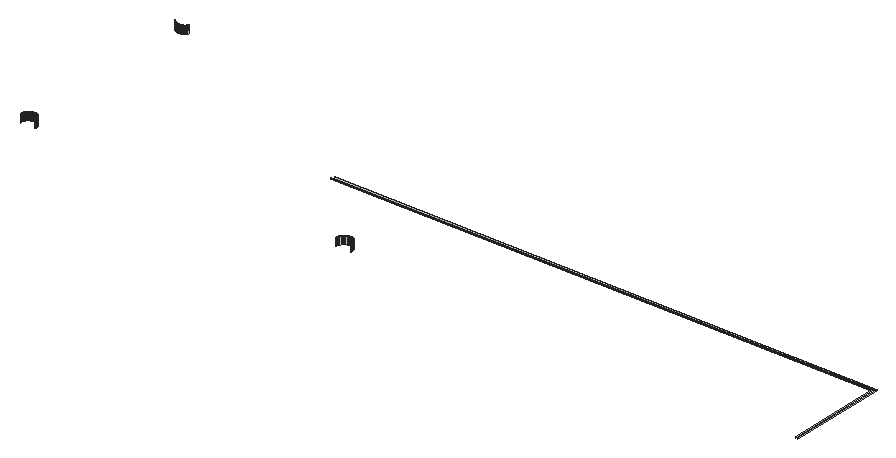
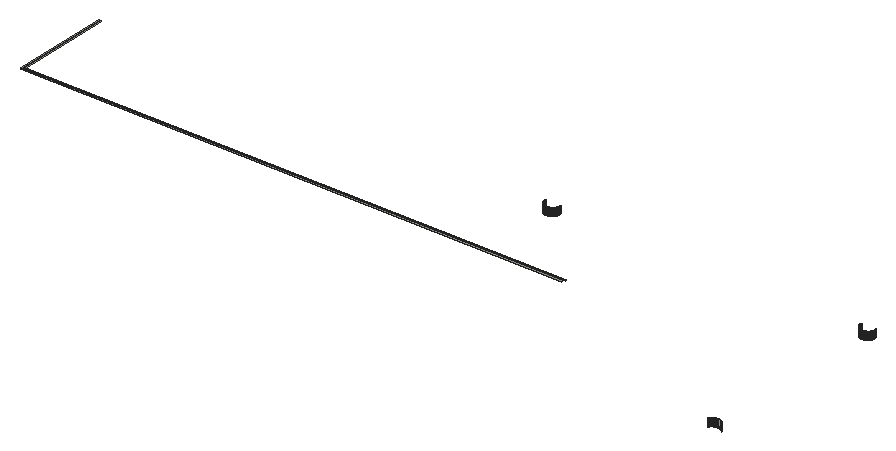
# SketchUp Ruby script. Lengths in inches.
U = 1.inch
M = Sketchup.active_model
def pt(a) = Geom::Point3d.new(a.map { |v| v * U })
def face(e, loops, mat)
  f = e.add_face(loops[0].map { |a| pt(a) })
  loops[1..].each { |l| e.add_face(l.map { |a| pt(a) }).erase! }
  f.material = f.back_material = mat if mat
  f
end
# faces: each face lists its corners as indices into pts; further lists are holes
def faces(e, pts, list, mat = nil) = list.each { |f| face(e, (f[0].is_a?(Array) ? f : [f]).map { |l| l.map { |i| pts[i] } }, mat) }
# xy, xz, yz: faces in a plane at the given z, y or x. An outline is a flat list of corners, or four numbers for a rectangle; further outlines are holes
def ring(l) = l.size == 4 ? [[l[0], l[1]], [l[2], l[1]], [l[2], l[3]], [l[0], l[3]]] : l.each_slice(2).to_a
def flat(e, list, mat, &to3) = list.each { |f| face(e, (f[0].is_a?(Array) ? f : [f]).map { |l| ring(l).map { |u, v| to3.(u, v) } }, mat) }
def xy(e, z, list, mat = nil) = flat(e, list, mat) { |x, y| [x, y, z] }
def xz(e, y, list, mat = nil) = flat(e, list, mat) { |x, z| [x, y, z] }
def yz(e, x, list, mat = nil) = flat(e, list, mat) { |y, z| [x, y, z] }
def lines(e, pts, list) = list.each { |a, b| e.add_line(pt(pts[a]), pt(pts[b])) }
# prism: a flat outline (further loops are holes) pulled along v
def prism(e, loops, v, mat = nil)
  f = face(e, loops, mat); d = Geom::Vector3d.new(v.map { |x| x * U })
  f.pushpull(f.normal.samedirection?(d) ? d.length : -d.length)
end
def box(e, o, s, mat = nil) = prism(e, [[o, [o[0] + s[0], o[1], o[2]], [o[0] + s[0], o[1] + s[1], o[2]], [o[0], o[1] + s[1], o[2]]]], [0, 0, s[2]], mat)
def at(x, y, z, deg = 0) = Geom::Transformation.translation(pt([x, y, z])) * Geom::Transformation.rotation(ORIGIN, Z_AXIS, deg.degrees)
def axes(o, x, y, z) = Geom::Transformation.new([*x, 0, *y, 0, *z, 0, *pt(o).to_a, 1])
def part(name) = M.definitions.add(name)
# library, detail: a bought-in or finely detailed component or shape, given as its bounding box
def library(name, o, s) = part(name).tap { |d| box(d.entities, o, s) }
def detail(e, o, s) = box(e.add_group.entities, o, s)
def put(e, d, t, mat = nil) = e.add_instance(d, t).tap { |i| i.material = mat if mat }
def group(e, t, mat = nil) = e.add_group.tap { |g| g.transformation = t; g.material = mat if mat }.entities
root = M.entities
M.materials.add("0027 AP L140 CRUSHED ICE").color = [241, 233, 217]
xz(root,261,[[59.84,120,59.92,123],[59.92,120,60,123],[60,120,60.08,123],[60.08,120,60.16,123],[185.84,120,185.92,123],
  [185.92,120,186,123],[186,120,186.08,123],[186.08,120,186.16,123]],"0027 AP L140 CRUSHED ICE")
xz(root,290,[[155,120,371,120.5]],"0027 AP L140 CRUSHED ICE")
xz(root,291,[[156,120,372,120.5]],"0027 AP L140 CRUSHED ICE")
xz(root,333,[[59.84,120,59.92,123],[59.92,120,60,123],[60,120,60.08,123],[60.08,120,60.16,123]],"0027 AP L140 CRUSHED ICE")
yz(root,57,[[257.84,120,257.92,123],[257.92,120,258,123],[258,120,258.08,123],[258.08,120,258.16,123]],"0027 AP L140 CRUSHED ICE")
yz(root,63,[[257.84,120,257.92,123],[257.92,120,258,123],[258,120,258.08,123],[258.08,120,258.16,123]],"0027 AP L140 CRUSHED ICE")
yz(root,183,[[257.84,120,257.92,123],[257.92,120,258,123],[258,120,258.08,123],[258.08,120,258.16,123]],"0027 AP L140 CRUSHED ICE")
yz(root,189,[[257.84,120,257.92,123],[257.92,120,258,123],[258,120,258.08,123],[258.08,120,258.16,123]],"0027 AP L140 CRUSHED ICE")
yz(root,371,[[252,120,290,120.5]],"0027 AP L140 CRUSHED ICE")
yz(root,372,[[252,120,291,120.5]],"0027 AP L140 CRUSHED ICE")
p = [[62.98,257.6875,120],[62.97,257.61,120],[62.97,257.61,123],[62.98,257.6875,123],[57.02,257.6875,120],[57.01,257.76,120],
  [57.01,257.76,123],[57.02,257.6875,123],[62.99,257.76,120],[62.99,257.76,123],[183.02,257.6875,120],[183.01,257.76,120],
  [183.01,257.76,123],[183.02,257.6875,123],[188.99,257.76,120],[188.98,257.6875,120],[188.98,257.6875,123],[188.99,257.76,123],
  [57,257.84,120],[57,257.84,123],[63,257.84,120],[63,257.84,123],[183,257.84,120],[183,257.84,123],
  [189,257.84,120],[189,257.84,123],[57,258.16,120],[57.01,258.24,120],[57.01,258.24,123],[57,258.16,123],
  [57.02,258.3125,120],[57.02,258.3125,123],[62.99,258.24,120],[63,258.16,120],[63,258.16,123],[62.99,258.24,123],
  [62.98,258.3125,120],[62.98,258.3125,123],[183,258.16,120],[183.01,258.24,120],[183.01,258.24,123],[183,258.16,123],
  [183.02,258.3125,120],[183.02,258.3125,123],[188.99,258.24,120],[189,258.16,120],[189,258.16,123],[188.99,258.24,123],
  [188.98,258.3125,120],[188.98,258.3125,123],[57.03,258.39,120],[57.03,258.39,123],[62.97,258.39,120],[62.97,258.39,123],
  [183.03,258.39,120],[183.03,258.39,123],[188.97,258.39,120],[188.97,258.39,123],[57.04,258.47,120],[57.04,258.47,123],
  [62.96,258.47,120],[62.96,258.47,123],[183.04,258.47,120],[183.04,258.47,123],[188.96,258.47,120],[188.96,258.47,123],
  [57.05,258.55,120],[57.05,258.55,123],[57.07,258.625,120],[57.07,258.625,123],[62.95,258.55,120],[62.95,258.55,123],
  [62.93,258.625,120],[62.93,258.625,123],[183.05,258.55,120],[183.05,258.55,123],[183.07,258.625,120],[183.07,258.625,123],
  [188.95,258.55,120],[188.95,258.55,123],[188.93,258.625,120],[188.93,258.625,123],[57.08,258.7,120],[57.08,258.7,123],
  [62.92,258.7,120],[62.92,258.7,123],[183.08,258.7,120],[183.08,258.7,123],[188.92,258.7,120],[188.92,258.7,123],
  [57.1,258.78,120],[57.1,258.78,123],[62.9,258.78,120],[62.9,258.78,123],[183.1,258.78,120],[183.1,258.78,123],
  [188.9,258.78,120],[188.9,258.78,123],[57.125,258.85,120],[57.125,258.85,123],[62.875,258.85,120],[62.875,258.85,123],
  [183.125,258.85,120],[183.125,258.85,123],[188.875,258.85,120],[188.875,258.85,123],[57.15,258.93,120],[57.15,258.93,123],
  [57.17,259,120],[57.17,259,123],[62.83,259,120],[62.85,258.93,120],[62.85,258.93,123],[62.83,259,123],
  [183.15,258.93,120],[183.15,258.93,123],[183.17,259,120],[183.17,259,123],[188.83,259,120],[188.85,258.93,120],
  [188.85,258.93,123],[188.83,259,123],[57.2,259.08,120],[57.2,259.08,123],[62.8,259.08,120],[62.8,259.08,123],
  [183.2,259.08,120],[183.2,259.08,123],[188.8,259.08,120],[188.8,259.08,123],[57.23,259.15,120],[57.23,259.15,123],
  [57.26,259.22,120],[57.26,259.22,123],[62.74,259.22,120],[62.77,259.15,120],[62.77,259.15,123],[62.74,259.22,123],
  [183.23,259.15,120],[183.23,259.15,123],[183.26,259.22,120],[183.26,259.22,123],[188.74,259.22,120],[188.77,259.15,120],
  [188.77,259.15,123],[188.74,259.22,123],[57.29,259.29,120],[57.29,259.29,123],[62.71,259.29,120],[62.71,259.29,123],
  [183.29,259.29,120],[183.29,259.29,123],[188.71,259.29,120],[188.71,259.29,123],[57.33,259.36,120],[57.33,259.36,123],
  [62.67,259.36,120],[62.67,259.36,123],[183.33,259.36,120],[183.33,259.36,123],[188.67,259.36,120],[188.67,259.36,123],
  [57.36,259.43,120],[57.36,259.43,123],[57.4,259.5,120],[57.4,259.5,123],[62.64,259.43,120],[62.64,259.43,123],
  [62.6,259.5,120],[62.6,259.5,123],[183.36,259.43,120],[183.36,259.43,123],[183.4,259.5,120],[183.4,259.5,123],
  [188.64,259.43,120],[188.64,259.43,123],[188.6,259.5,120],[188.6,259.5,123],[57.44,259.57,120],[57.44,259.57,123],
  [62.56,259.57,120],[62.56,259.57,123],[183.44,259.57,120],[183.44,259.57,123],[188.56,259.57,120],[188.56,259.57,123],
  [57.48,259.63,120],[57.48,259.63,123],[57.53,259.7,120],[57.53,259.7,123],[62.52,259.63,120],[62.52,259.63,123],
  [62.47,259.7,120],[62.47,259.7,123],[183.48,259.63,120],[183.48,259.63,123],[183.53,259.7,120],[183.53,259.7,123],
  [188.52,259.63,120],[188.52,259.63,123],[188.47,259.7,120],[188.47,259.7,123],[57.57,259.76,120],[57.57,259.76,123],
  [62.43,259.76,120],[62.43,259.76,123],[183.57,259.76,120],[183.57,259.76,123],[188.43,259.76,120],[188.43,259.76,123],
  [57.62,259.83,120],[57.62,259.83,123],[57.67,259.89,120],[57.67,259.89,123],[62.33,259.89,120],[62.38,259.83,120],
  [62.38,259.83,123],[62.33,259.89,123],[183.62,259.83,120],[183.62,259.83,123],[183.67,259.89,120],[183.67,259.89,123],
  [188.33,259.89,120],[188.38,259.83,120],[188.38,259.83,123],[188.33,259.89,123],[57.72,259.95,120],[57.72,259.95,123],
  [57.77,260.01,120],[57.77,260.01,123],[62.23,260.01,120],[62.28,259.95,120],[62.28,259.95,123],[62.23,260.01,123],
  [183.72,259.95,120],[183.72,259.95,123],[183.77,260.01,120],[183.77,260.01,123],[188.23,260.01,120],[188.28,259.95,120],
  [188.28,259.95,123],[188.23,260.01,123],[57.82,260.07,120],[57.82,260.07,123],[62.18,260.07,120],[62.18,260.07,123],
  [183.82,260.07,120],[183.82,260.07,123],[188.18,260.07,120],[188.18,260.07,123],[57.88,260.12,120],[57.88,260.12,123],
  [57.93,260.18,120],[57.93,260.18,123],[62.12,260.12,120],[62.12,260.12,123],[62.07,260.18,120],[62.07,260.18,123],
  [183.88,260.12,120],[183.88,260.12,123],[183.93,260.18,120],[183.93,260.18,123],[188.12,260.12,120],[188.12,260.12,123],
  [188.07,260.18,120],[188.07,260.18,123],[57.99,260.23,120],[57.99,260.23,123],[58.05,260.28,120],[58.05,260.28,123],
  [61.95,260.28,120],[62.01,260.23,120],[62.01,260.23,123],[61.95,260.28,123],[183.99,260.23,120],[183.99,260.23,123],
  [184.05,260.28,120],[184.05,260.28,123],[187.95,260.28,120],[188.01,260.23,120],[188.01,260.23,123],[187.95,260.28,123],
  [58.11,260.33,120],[58.11,260.33,123],[58.17,260.38,120],[58.17,260.38,123],[61.83,260.38,120],[61.89,260.33,120],
  [61.89,260.33,123],[61.83,260.38,123],[184.11,260.33,120],[184.11,260.33,123],[184.17,260.38,120],[184.17,260.38,123],
  [187.83,260.38,120],[187.89,260.33,120],[187.89,260.33,123],[187.83,260.38,123],[58.24,260.43,120],[58.24,260.43,123],
  [58.3,260.47,120],[58.3,260.47,123],[61.7,260.47,120],[61.76,260.43,120],[61.76,260.43,123],[61.7,260.47,123],
  [184.24,260.43,120],[184.24,260.43,123],[184.3,260.47,120],[184.3,260.47,123],[187.7,260.47,120],[187.76,260.43,120],
  [187.76,260.43,123],[187.7,260.47,123],[58.37,260.52,120],[58.37,260.52,123],[58.43,260.56,120],[58.43,260.56,123],
  [61.63,260.52,120],[61.63,260.52,123],[61.57,260.56,120],[61.57,260.56,123],[184.37,260.52,120],[184.37,260.52,123],
  [184.43,260.56,120],[184.43,260.56,123],[187.63,260.52,120],[187.63,260.52,123],[187.57,260.56,120],[187.57,260.56,123],
  [58.5,260.6,120],[58.5,260.6,123],[58.57,260.64,120],[58.57,260.64,123],[58.64,260.67,120],[58.64,260.67,123],
  [61.43,260.64,120],[61.5,260.6,120],[61.5,260.6,123],[61.43,260.64,123],[61.36,260.67,120],[61.36,260.67,123],
  [184.5,260.6,120],[184.5,260.6,123],[184.57,260.64,120],[184.57,260.64,123],[184.64,260.67,120],[184.64,260.67,123],
  [187.43,260.64,120],[187.5,260.6,120],[187.5,260.6,123],[187.43,260.64,123],[187.36,260.67,120],[187.36,260.67,123],
  [58.71,260.71,120],[58.71,260.71,123],[58.78,260.74,120],[58.78,260.74,123],[58.85,260.77,120],[58.85,260.77,123],
  [61.15,260.77,120],[61.22,260.74,120],[61.22,260.74,123],[61.15,260.77,123],[61.29,260.71,120],[61.29,260.71,123],
  [184.71,260.71,120],[184.71,260.71,123],[184.78,260.74,120],[184.78,260.74,123],[184.85,260.77,120],[184.85,260.77,123],
  [187.15,260.77,120],[187.22,260.74,120],[187.22,260.74,123],[187.15,260.77,123],[187.29,260.71,120],[187.29,260.71,123],
  [58.92,260.8,120],[58.92,260.8,123],[59,260.83,120],[59,260.83,123],[59.07,260.85,120],[59.07,260.85,123],
  [60.93,260.85,120],[61,260.83,120],[61,260.83,123],[60.93,260.85,123],[61.08,260.8,120],[61.08,260.8,123],
  [184.92,260.8,120],[184.92,260.8,123],[185,260.83,120],[185,260.83,123],[185.07,260.85,120],[185.07,260.85,123],
  [186.93,260.85,120],[187,260.83,120],[187,260.83,123],[186.93,260.85,123],[187.08,260.8,120],[187.08,260.8,123],
  [59.15,260.875,120],[59.15,260.875,123],[59.22,260.9,120],[59.22,260.9,123],[59.3,260.92,120],[59.3,260.92,123],
  [59.375,260.93,120],[59.375,260.93,123],[59.45,260.95,120],[59.45,260.95,123],[59.53,260.96,120],[59.53,260.96,123],
  [60.55,260.95,120],[60.625,260.93,120],[60.625,260.93,123],[60.55,260.95,123],[60.47,260.96,120],[60.47,260.96,123],
  [60.7,260.92,120],[60.7,260.92,123],[60.78,260.9,120],[60.78,260.9,123],[60.85,260.875,120],[60.85,260.875,123],
  [185.15,260.875,120],[185.15,260.875,123],[185.22,260.9,120],[185.22,260.9,123],[185.3,260.92,120],[185.3,260.92,123],
  [185.375,260.93,120],[185.375,260.93,123],[185.45,260.95,120],[185.45,260.95,123],[185.53,260.96,120],[185.53,260.96,123],
  [186.55,260.95,120],[186.625,260.93,120],[186.625,260.93,123],[186.55,260.95,123],[186.47,260.96,120],[186.47,260.96,123],
  [186.7,260.92,120],[186.7,260.92,123],[186.78,260.9,120],[186.78,260.9,123],[186.85,260.875,120],[186.85,260.875,123],
  [59.61,260.97,120],[59.61,260.97,123],[59.6875,260.98,120],[59.6875,260.98,123],[59.76,260.99,120],[59.76,260.99,123],
  [59.84,261,120],[59.84,261,123],[60.24,260.99,120],[60.3125,260.98,120],[60.3125,260.98,123],[60.24,260.99,123],
  [60.16,261,120],[60.16,261,123],[60.39,260.97,120],[60.39,260.97,123],[185.61,260.97,120],[185.61,260.97,123],
  [185.6875,260.98,120],[185.6875,260.98,123],[185.76,260.99,120],[185.76,260.99,123],[185.84,261,120],[185.84,261,123],
  [186.24,260.99,120],[186.3125,260.98,120],[186.3125,260.98,123],[186.24,260.99,123],[186.16,261,120],[186.16,261,123],
  [186.39,260.97,120],[186.39,260.97,123],[59.61,333.03,120],[59.53,333.04,120],[59.53,333.04,123],[59.61,333.03,123],
  [59.45,333.05,120],[59.45,333.05,123],[59.6875,333.02,120],[59.6875,333.02,123],[59.76,333.01,120],[59.76,333.01,123],
  [59.84,333,120],[59.84,333,123],[60.24,333.01,120],[60.16,333,120],[60.16,333,123],[60.24,333.01,123],
  [60.3125,333.02,120],[60.3125,333.02,123],[60.39,333.03,120],[60.39,333.03,123],[60.47,333.04,120],[60.47,333.04,123],
  [60.55,333.05,120],[60.55,333.05,123],[59.07,333.15,120],[59,333.17,120],[59,333.17,123],[59.07,333.15,123],
  [59.22,333.1,120],[59.15,333.125,120],[59.15,333.125,123],[59.22,333.1,123],[59.3,333.08,120],[59.3,333.08,123],
  [59.375,333.07,120],[59.375,333.07,123],[60.625,333.07,120],[60.625,333.07,123],[60.7,333.08,120],[60.7,333.08,123],
  [60.78,333.1,120],[60.78,333.1,123],[60.85,333.125,120],[60.85,333.125,123],[60.93,333.15,120],[60.93,333.15,123],
  [61,333.17,120],[61,333.17,123],[58.85,333.23,120],[58.78,333.26,120],[58.78,333.26,123],[58.85,333.23,123],
  [58.92,333.2,120],[58.92,333.2,123],[61.08,333.2,120],[61.08,333.2,123],[61.15,333.23,120],[61.15,333.23,123],
  [61.22,333.26,120],[61.22,333.26,123],[58.71,333.29,120],[58.64,333.33,120],[58.64,333.33,123],[58.71,333.29,123],
  [58.57,333.36,120],[58.57,333.36,123],[61.29,333.29,120],[61.29,333.29,123],[61.36,333.33,120],[61.36,333.33,123],
  [61.43,333.36,120],[61.43,333.36,123],[58.5,333.4,120],[58.43,333.44,120],[58.43,333.44,123],[58.5,333.4,123],
  [58.37,333.48,120],[58.37,333.48,123],[61.5,333.4,120],[61.5,333.4,123],[61.57,333.44,120],[61.57,333.44,123],
  [61.63,333.48,120],[61.63,333.48,123],[58.3,333.53,120],[58.24,333.57,120],[58.24,333.57,123],[58.3,333.53,123],
  [61.7,333.53,120],[61.7,333.53,123],[61.76,333.57,120],[61.76,333.57,123],[58.17,333.62,120],[58.11,333.67,120],
  [58.11,333.67,123],[58.17,333.62,123],[61.83,333.62,120],[61.83,333.62,123],[61.89,333.67,120],[61.89,333.67,123],
  [58.05,333.72,120],[57.99,333.77,120],[57.99,333.77,123],[58.05,333.72,123],[61.95,333.72,120],[61.95,333.72,123],
  [62.01,333.77,120],[62.01,333.77,123],[57.93,333.82,120],[57.93,333.82,123],[57.88,333.88,120],[57.88,333.88,123],
  [62.07,333.82,120],[62.07,333.82,123],[62.12,333.88,120],[62.12,333.88,123],[57.82,333.93,120],[57.82,333.93,123],
  [57.77,333.99,120],[57.77,333.99,123],[62.18,333.93,120],[62.18,333.93,123],[62.23,333.99,120],[62.23,333.99,123],
  [57.72,334.05,120],[57.72,334.05,123],[62.28,334.05,120],[62.28,334.05,123],[57.67,334.11,120],[57.62,334.17,120],
  [57.62,334.17,123],[57.67,334.11,123],[62.33,334.11,120],[62.33,334.11,123],[62.38,334.17,120],[62.38,334.17,123],
  [57.57,334.24,120],[57.53,334.3,120],[57.53,334.3,123],[57.57,334.24,123],[62.43,334.24,120],[62.43,334.24,123],
  [62.47,334.3,120],[62.47,334.3,123],[57.48,334.37,120],[57.48,334.37,123],[62.52,334.37,120],[62.52,334.37,123],
  [57.44,334.43,120],[57.44,334.43,123],[57.4,334.5,120],[57.4,334.5,123],[62.56,334.43,120],[62.56,334.43,123],
  [62.6,334.5,120],[62.6,334.5,123],[57.36,334.57,120],[57.36,334.57,123],[62.64,334.57,120],[62.64,334.57,123]]
faces(root,p,[[0,1,2,3],[4,5,6,7],[8,0,3,9],[10,11,12,13],[14,15,16,17],[5,18,19,6],[20,8,9,21],[11,22,23,12],
  [24,14,17,25],[26,27,28,29],[27,30,31,28],[32,33,34,35],[36,32,35,37],[38,39,40,41],[39,42,43,40],[44,45,46,47],
  [48,44,47,49],[30,50,51,31],[52,36,37,53],[42,54,55,43],[56,48,49,57],[50,58,59,51],[60,52,53,61],[54,62,63,55],
  [64,56,57,65],[58,66,67,59],[66,68,69,67],[70,60,61,71],[72,70,71,73],[62,74,75,63],[74,76,77,75],[78,64,65,79],
  [80,78,79,81],[68,82,83,69],[84,72,73,85],[76,86,87,77],[88,80,81,89],[82,90,91,83],[92,84,85,93],[86,94,95,87],
  [96,88,89,97],[90,98,99,91],[100,92,93,101],[94,102,103,95],[104,96,97,105],[98,106,107,99],[106,108,109,107],[110,111,112,113],
  [111,100,101,112],[102,114,115,103],[114,116,117,115],[118,119,120,121],[119,104,105,120],[108,122,123,109],[124,110,113,125],[116,126,127,117],
  [128,118,121,129],[122,130,131,123],[130,132,133,131],[134,135,136,137],[135,124,125,136],[126,138,139,127],[138,140,141,139],[142,143,144,145],
  [143,128,129,144],[132,146,147,133],[148,134,137,149],[140,150,151,141],[152,142,145,153],[146,154,155,147],[156,148,149,157],[150,158,159,151],
  [160,152,153,161],[154,162,163,155],[162,164,165,163],[166,156,157,167],[168,166,167,169],[158,170,171,159],[170,172,173,171],[174,160,161,175],
  [176,174,175,177],[164,178,179,165],[180,168,169,181],[172,182,183,173],[184,176,177,185],[178,186,187,179],[186,188,189,187],[190,180,181,191],
  [192,190,191,193],[182,194,195,183],[194,196,197,195],[198,184,185,199],[200,198,199,201],[188,202,203,189],[204,192,193,205],[196,206,207,197],
  [208,200,201,209],[202,210,211,203],[210,212,213,211],[214,215,216,217],[215,204,205,216],[206,218,219,207],[218,220,221,219],[222,223,224,225],
  [223,208,209,224],[212,226,227,213],[226,228,229,227],[230,231,232,233],[231,214,217,232],[220,234,235,221],[234,236,237,235],[238,239,240,241],
  [239,222,225,240],[228,242,243,229],[244,230,233,245],[236,246,247,237],[248,238,241,249],[242,250,251,243],[250,252,253,251],[254,244,245,255],
  [256,254,255,257],[246,258,259,247],[258,260,261,259],[262,248,249,263],[264,262,263,265],[252,266,267,253],[266,268,269,267],[270,271,272,273],
  [271,256,257,272],[260,274,275,261],[274,276,277,275],[278,279,280,281],[279,264,265,280],[268,282,283,269],[282,284,285,283],[286,287,288,289],
  [287,270,273,288],[276,290,291,277],[290,292,293,291],[294,295,296,297],[295,278,281,296],[284,298,299,285],[298,300,301,299],[302,303,304,305],
  [303,286,289,304],[292,306,307,293],[306,308,309,307],[310,311,312,313],[311,294,297,312],[300,314,315,301],[314,316,317,315],[318,302,305,319],
  [320,318,319,321],[308,322,323,309],[322,324,325,323],[326,310,313,327],[328,326,327,329],[316,330,331,317],[330,332,333,331],[332,334,335,333],
  [336,337,338,339],[340,336,339,341],[337,320,321,338],[324,342,343,325],[342,344,345,343],[344,346,347,345],[348,349,350,351],[352,348,351,353],
  [349,328,329,350],[334,354,355,335],[354,356,357,355],[356,358,359,357],[360,361,362,363],[361,364,365,362],[364,340,341,365],[346,366,367,347],
  [366,368,369,367],[368,370,371,369],[372,373,374,375],[373,376,377,374],[376,352,353,377],[358,378,379,359],[378,380,381,379],[380,382,383,381],
  [384,385,386,387],[385,388,389,386],[388,360,363,389],[370,390,391,371],[390,392,393,391],[392,394,395,393],[396,397,398,399],[397,400,401,398],
  [400,372,375,401],[382,402,403,383],[402,404,405,403],[404,406,407,405],[406,408,409,407],[408,410,411,409],[410,412,413,411],[414,415,416,417],
  [418,414,417,419],[415,420,421,416],[420,422,423,421],[422,424,425,423],[424,384,387,425],[394,426,427,395],[426,428,429,427],[428,430,431,429],
  [430,432,433,431],[432,434,435,433],[434,436,437,435],[438,439,440,441],[442,438,441,443],[439,444,445,440],[444,446,447,445],[446,448,449,447],
  [448,396,399,449],[412,450,451,413],[450,452,453,451],[452,454,455,453],[454,456,457,455],[458,459,460,461],[462,458,461,463],[459,464,465,460],
  [464,418,419,465],[436,466,467,437],[466,468,469,467],[468,470,471,469],[470,472,473,471],[474,475,476,477],[478,474,477,479],[475,480,481,476],
  [480,442,443,481],[482,483,484,485],[483,486,487,484],[488,482,485,489],[490,488,489,491],[492,490,491,493],[494,495,496,497],[498,494,497,499],
  [500,498,499,501],[502,500,501,503],[504,502,503,505],[506,507,508,509],[510,511,512,513],[511,506,509,512],[514,510,513,515],[516,514,515,517],
  [486,516,517,487],[518,504,505,519],[520,518,519,521],[522,520,521,523],[524,522,523,525],[526,524,525,527],[528,526,527,529],[530,531,532,533],
  [507,534,535,508],[534,530,533,535],[536,528,529,537],[538,536,537,539],[540,538,539,541],[542,543,544,545],[543,546,547,544],[531,542,545,532],
  [548,540,541,549],[550,548,549,551],[552,550,551,553],[554,555,556,557],[555,558,559,556],[546,554,557,547],[560,552,553,561],[562,560,561,563],
  [564,562,563,565],[566,567,568,569],[558,566,569,559],[570,564,565,571],[572,570,571,573],[574,575,576,577],[567,574,577,568],[578,572,573,579],
  [580,578,579,581],[582,583,584,585],[575,582,585,576],[586,580,581,587],[588,586,587,589],[583,590,591,584],[590,592,593,591],[594,588,589,595],
  [596,594,595,597],[592,598,599,593],[598,600,601,599],[602,596,597,603],[604,602,603,605],[600,606,607,601],[608,604,605,609],[610,611,612,613],
  [606,610,613,607],[614,608,609,615],[616,614,615,617],[618,619,620,621],[611,618,621,612],[622,616,617,623],[624,622,623,625],[619,626,627,620],
  [628,624,625,629],[626,630,631,627],[630,632,633,631],[634,628,629,635],[636,634,635,637],[632,638,639,633],[640,636,637,641]],"0027 AP L140 CRUSHED ICE")
